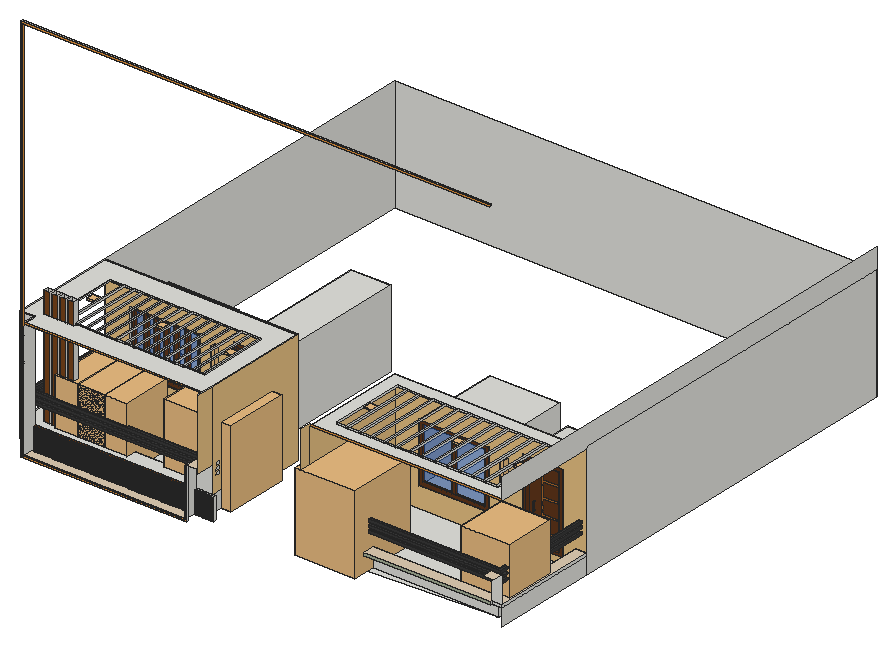
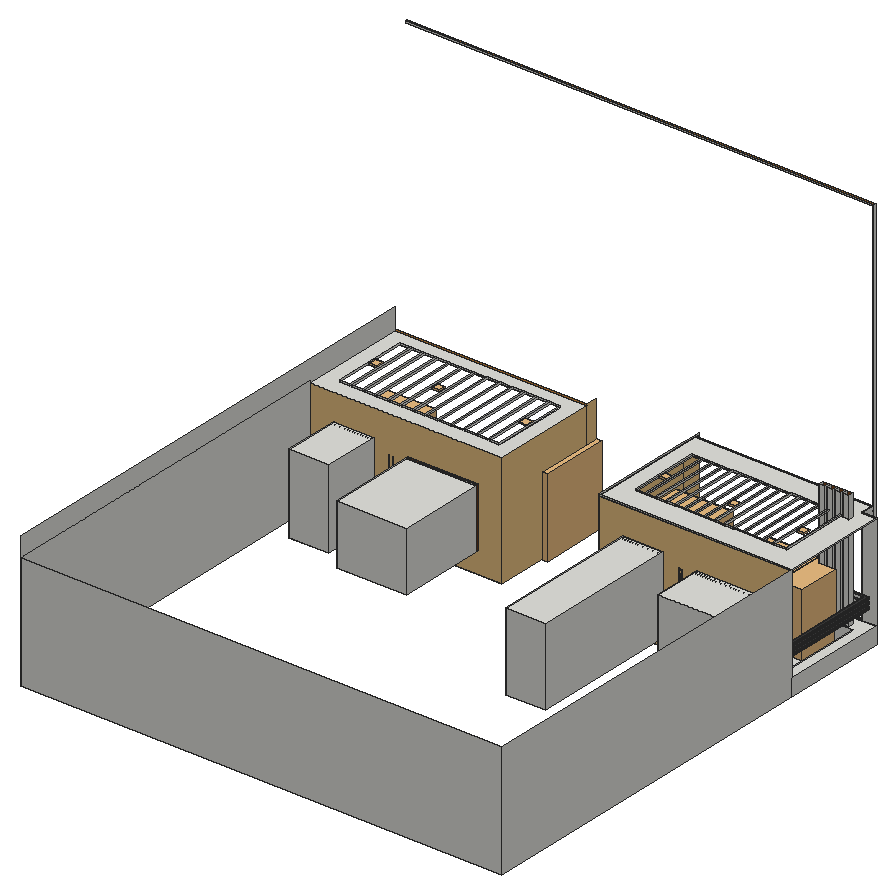
# SketchUp Ruby script. Lengths in inches.
U = 1.inch
M = Sketchup.active_model
def pt(a) = Geom::Point3d.new(a.map { |v| v * U })
def face(e, loops, mat)
  f = e.add_face(loops[0].map { |a| pt(a) })
  loops[1..].each { |l| e.add_face(l.map { |a| pt(a) }).erase! }
  f.material = f.back_material = mat if mat
  f
end
# faces: each face lists its corners as indices into pts; further lists are holes
def faces(e, pts, list, mat = nil) = list.each { |f| face(e, (f[0].is_a?(Array) ? f : [f]).map { |l| l.map { |i| pts[i] } }, mat) }
# xy, xz, yz: faces in a plane at the given z, y or x. An outline is a flat list of corners, or four numbers for a rectangle; further outlines are holes
def ring(l) = l.size == 4 ? [[l[0], l[1]], [l[2], l[1]], [l[2], l[3]], [l[0], l[3]]] : l.each_slice(2).to_a
def flat(e, list, mat, &to3) = list.each { |f| face(e, (f[0].is_a?(Array) ? f : [f]).map { |l| ring(l).map { |u, v| to3.(u, v) } }, mat) }
def xy(e, z, list, mat = nil) = flat(e, list, mat) { |x, y| [x, y, z] }
def xz(e, y, list, mat = nil) = flat(e, list, mat) { |x, z| [x, y, z] }
def yz(e, x, list, mat = nil) = flat(e, list, mat) { |y, z| [x, y, z] }
def lines(e, pts, list) = list.each { |a, b| e.add_line(pt(pts[a]), pt(pts[b])) }
# prism: a flat outline (further loops are holes) pulled along v
def prism(e, loops, v, mat = nil)
  f = face(e, loops, mat); d = Geom::Vector3d.new(v.map { |x| x * U })
  f.pushpull(f.normal.samedirection?(d) ? d.length : -d.length)
end
def box(e, o, s, mat = nil) = prism(e, [[o, [o[0] + s[0], o[1], o[2]], [o[0] + s[0], o[1] + s[1], o[2]], [o[0], o[1] + s[1], o[2]]]], [0, 0, s[2]], mat)
def at(x, y, z, deg = 0) = Geom::Transformation.translation(pt([x, y, z])) * Geom::Transformation.rotation(ORIGIN, Z_AXIS, deg.degrees)
def axes(o, x, y, z) = Geom::Transformation.new([*x, 0, *y, 0, *z, 0, *pt(o).to_a, 1])
def part(name) = M.definitions.add(name)
# library, detail: a bought-in or finely detailed component or shape, given as its bounding box
def library(name, o, s) = part(name).tap { |d| box(d.entities, o, s) }
def detail(e, o, s) = box(e.add_group.entities, o, s)
def put(e, d, t, mat = nil) = e.add_instance(d, t).tap { |i| i.material = mat if mat }
def group(e, t, mat = nil) = e.add_group.tap { |g| g.transformation = t; g.material = mat if mat }.entities
root = M.entities
M.materials.add("Generic\#1").color = [121, 68, 27]
M.materials.add("Generic\#4").color = [232, 149, 60]
M.materials.add("Generic\#5").color = [233, 194, 132]
M.materials.add("Generic\#6").color = [223, 205, 179]
M.materials.add("Generic\#8").color = [168, 180, 155]
M.materials.add("[Color M05]").color = [114, 114, 114]
M.materials.add("[Color M07]").color = [58, 58, 58]
M.materials.add("[Translucent Glass Blue]").color = [28, 83, 181]
M.materials["[Translucent Glass Blue]"].alpha = 0.5
M.materials.add("[Wood Bamboo]").color = [177, 105, 43]
M.materials.add("[Wood Cherry Original]").color = [96, 54, 26]
c1 = part("Group\#9")
xy(c1.entities,22.76,[[0,0,2,3]])
xz(c1.entities,0,[[0,0,2,22.76]])
yz(c1.entities,0,[[0,0,3,22.76]])
yz(c1.entities,2,[[0,0,3,22.76]])
c2 = library("Plant",[-27.84,-31.84,-1.26],[68.28,70.82,154.38])
c3 = library("Plant+2 (1)",[-9.13,-9.52,0],[51.76,51.77,66.88])
c4 = library("Flora+17",[-57.52,158.6,-38.64],[66.99,62.88,77.28])
c5 = part("Group\#5")
xy(c5.entities,0,[[0,0,41.8125,3.4375]],"[Wood Cherry Original]")
xy(c5.entities,3.53,[[3.53,0,38.28,3.4375]],"[Wood Cherry Original]")
xy(c5.entities,31.39,[[9.28,1.32,9.97,3.4375]])
xy(c5.entities,32.05,[[9.29,1.98,9.98,3.4375]],"[Color M05]")
xy(c5.entities,39.77,[[9.29,1.98,9.98,3.4375]])
xy(c5.entities,40.43,[[9.28,1.32,9.97,3.4375]],"[Color M05]")
xy(c5.entities,79.47,[[3.53,0,38.28,3.4375]],"[Wood Cherry Original]")
xy(c5.entities,83,[[0,0,41.8125,3.4375]],"[Wood Cherry Original]")
xz(c5.entities,0,[[[0,0,41.8125,83],[3.53,3.53,38.28,79.47]]],"[Wood Cherry Original]")
xz(c5.entities,1.32,[[9.28,31.39,9.97,40.43]],"[Color M05]")
xz(c5.entities,1.98,[[9.29,32.05,9.98,39.77]],"[Color M05]")
xz(c5.entities,3.4375,[[9.29,39.77,9.28,40.43,9.97,40.43,9.98,39.77]])
xz(c5.entities,3.4375,[[16.22,3.53,17.74,3.53,17.74,13.29,38.28,13.29,38.28,15.09,17.74,15.09,17.74,29.41,38.28,29.41,38.28,31.22,17.74,31.22,17.74,45.54,38.28,45.54,38.28,47.34,17.74,47.34,17.74,61.66,38.28,61.66,38.28,63.47,17.74,63.47,17.74,79.47,16.22,79.47]],"[Wood Bamboo]")
xz(c5.entities,3.4375,[[[0,0,41.8125,83],[3.53,3.53,38.28,79.47]],[[3.53,3.53,16.22,79.47],[9.29,39.77,9.28,40.43,9.97,40.43,9.98,39.77],[9.28,31.39,9.29,32.05,9.98,32.05,9.97,31.39]],[17.74,3.53,38.28,13.29],[17.74,15.09,38.28,29.41],[17.74,31.22,38.28,45.54],
  [17.74,47.34,38.28,61.66],[17.74,63.47,38.28,79.47]],"[Wood Cherry Original]")
yz(c5.entities,0,[[0,0,3.4375,83]],"[Wood Cherry Original]")
yz(c5.entities,3.53,[[0,3.53,3.4375,79.47]],"[Wood Cherry Original]")
yz(c5.entities,38.28,[[0,3.53,3.4375,79.47]],"[Wood Cherry Original]")
yz(c5.entities,41.8125,[[0,0,3.4375,83]],"[Wood Cherry Original]")
p = [[9.28,1.32,40.43],[9.29,1.98,39.77],[9.29,1.98,32.05],[9.28,1.32,31.39],[9.29,3.4375,32.05],[9.28,3.4375,31.39],
  [9.98,1.98,39.77],[9.97,1.32,40.43],[9.97,1.32,31.39],[9.98,1.98,32.05],[9.97,3.4375,31.39],[9.98,3.4375,32.05],
  [9.28,3.4375,40.43],[9.29,3.4375,39.77],[9.98,3.4375,39.77],[9.97,3.4375,40.43],[9.625,3.4375,40.13],[9.625,1.625,40.13],
  [9.625,1.625,31.69],[9.625,3.4375,31.69]]
faces(c5.entities,p,[[0,1,2,3],[3,2,4,5],[6,7,8,9],[9,8,10,11],[12,13,1,0],[14,15,7,6]],"[Color M05]")
lines(c5.entities,p,[[16,17],[18,19],[17,18]])
c6 = part("Group\#3")
xy(c6.entities,0,[[0,0,81.86,2.5]],"[Wood Cherry Original]")
xy(c6.entities,4.12,[[4.12,0,13.68,2.5],[13.68,0,18.93,2.5],[18.93,0,25.68,2.5],[25.68,0,30.93,2.5],[30.93,0,37.68,2.5],
  [37.68,0,42.93,2.5],[42.93,0,49.68,2.5],[49.68,0,54.93,2.5],[54.93,0,61.68,2.5],[61.68,0,66.93,2.5],
  [66.93,0,77.74,2.5]],"[Wood Cherry Original]")
xy(c6.entities,66.49,[[4.12,0,13.68,2.5],[13.68,0,18.93,2.5],[18.93,0,25.68,2.5],[25.68,0,30.93,2.5],[30.93,0,37.68,2.5],
  [37.68,0,42.93,2.5],[42.93,0,49.68,2.5],[49.68,0,54.93,2.5],[54.93,0,61.68,2.5],[61.68,0,66.93,2.5],
  [66.93,0,77.74,2.5]],"[Wood Cherry Original]")
xy(c6.entities,70.61,[[0,0,81.86,2.5]],"[Wood Cherry Original]")
xz(c6.entities,0,[[[0,0,81.86,70.61],[4.12,4.12,77.74,66.49]],[13.68,4.12,18.93,66.49],[25.68,4.12,30.93,66.49],[37.68,4.12,42.93,66.49],[49.68,4.12,54.93,66.49],
  [61.68,4.12,66.93,66.49]],"[Wood Cherry Original]")
xz(c6.entities,2.5,[[4.12,4.12,13.68,66.49],[18.93,4.12,25.68,66.49],[30.93,4.12,37.68,66.49],[42.93,4.12,49.68,66.49],[54.93,4.12,61.68,66.49],
  [66.93,4.12,77.74,66.49]],"[Translucent Glass Blue]")
xz(c6.entities,2.5,[[[0,0,81.86,70.61],[4.12,4.12,77.74,66.49]]],"[Wood Cherry Original]")
yz(c6.entities,0,[[0,0,2.5,70.61]],"[Wood Cherry Original]")
yz(c6.entities,4.12,[[0,4.12,2.5,66.49]],"[Wood Cherry Original]")
yz(c6.entities,13.68,[[0,4.12,2.5,66.49]],"[Wood Cherry Original]")
yz(c6.entities,18.93,[[0,4.12,2.5,66.49]],"[Wood Cherry Original]")
yz(c6.entities,25.68,[[0,4.12,2.5,66.49]],"[Wood Cherry Original]")
yz(c6.entities,30.93,[[0,4.12,2.5,66.49]],"[Wood Cherry Original]")
yz(c6.entities,37.68,[[0,4.12,2.5,66.49]],"[Wood Cherry Original]")
yz(c6.entities,42.93,[[0,4.12,2.5,66.49]],"[Wood Cherry Original]")
yz(c6.entities,49.68,[[0,4.12,2.5,66.49]],"[Wood Cherry Original]")
yz(c6.entities,54.93,[[0,4.12,2.5,66.49]],"[Wood Cherry Original]")
yz(c6.entities,61.68,[[0,4.12,2.5,66.49]],"[Wood Cherry Original]")
yz(c6.entities,66.93,[[0,4.12,2.5,66.49]],"[Wood Cherry Original]")
yz(c6.entities,77.74,[[0,4.12,2.5,66.49]],"[Wood Cherry Original]")
yz(c6.entities,81.86,[[0,0,2.5,70.61]],"[Wood Cherry Original]")
c7 = part("Group\#4")
xy(c7.entities,0,[[0,0,73.625,2.0625]],"[Wood Cherry Original]")
xy(c7.entities,3.98,[[35.0625,0,38.75,2.0625]])
xy(c7.entities,3.98,[[3.98,0,35.0625,2.0625],[38.75,0,69.64,2.0625]],"[Wood Cherry Original]")
xy(c7.entities,58.39,[[35.0625,0,38.75,2.0625]])
xy(c7.entities,58.39,[[3.98,0,35.0625,2.0625],[38.75,0,69.64,2.0625]],"[Wood Cherry Original]")
xy(c7.entities,62.375,[[0,0,73.625,2.0625]],"[Wood Cherry Original]")
xz(c7.entities,0,[[[0,0,73.625,62.375],[3.98,3.98,69.64,58.39]],[35.0625,3.98,38.75,58.39]],"[Wood Cherry Original]")
xz(c7.entities,2.0625,[[[0,0,73.625,62.375],[3.98,3.98,69.64,58.39]]])
xz(c7.entities,2.0625,[[3.98,3.98,35.0625,58.39],[38.75,3.98,69.64,58.39]],"[Translucent Glass Blue]")
yz(c7.entities,0,[[0,0,2.0625,62.375]],"[Wood Cherry Original]")
yz(c7.entities,3.98,[[0,3.98,2.0625,58.39]],"[Wood Cherry Original]")
yz(c7.entities,35.0625,[[0,3.98,2.0625,58.39]],"[Wood Cherry Original]")
yz(c7.entities,38.75,[[0,3.98,2.0625,58.39]],"[Wood Cherry Original]")
yz(c7.entities,69.64,[[0,3.98,2.0625,58.39]],"[Wood Cherry Original]")
yz(c7.entities,73.625,[[0,0,2.0625,62.375]],"[Wood Cherry Original]")
c8 = library("Lamp Wall Outdoor 94-02",[-1.89,-4.65,-3.17],[3.78,4.65,6.35])
c9 = library("Tlon Light 450 Ceiling 152 006",[-8.86,-8.86,-3.78],[17.72,17.72,3.56])
xy(root,133.9375,[[15.3125,39.5,189,41]])
xy(root,135.68,[[18.375,51.5625,20.375,54.5625]])
xy(root,135.68,[[17.125,39.5,187.19,41]],"Generic\#4")
xy(root,135.68,[[17.125,41,187.19,41,187.19,54.5625,20.375,54.5625,20.375,51.5625,18.375,51.5625,18.375,54.5625,17.125,54.5625]],"Generic\#6")
xy(root,140.875,[[306.09,54.5625,306.09,65.5625,496.1875,65.5625],[306.09,65.5625,496.1875,166.1875],[496.1875,65.5625,496.1875,166.1875,507.875,166.1875],[13.4375,71.3125,204.09,166.1875]])
xy(root,148.11,[[440.99,166.1875,482.8,225.0625]])
xy(root,148.65,[[137.36,166.1875,179.17,320.375]])
xy(root,158.4375,[[316.59,52.5625,318.59,54.5625],[318.59,52.5625,497.875,54.5625],[[2.3125,54.5625,204.09,54.5625,204.09,71.3125,13.4375,71.3125,13.4375,166.1875,2.3125,166.1875],[36.28,64.07,42.47,69.2],[27.85,64.07,34.03,69.2],[44.72,64.07,50.91,69.2],[19.41,64.07,25.6,69.2]],[306.09,54.5625,306.09,65.5625,496.1875,65.5625,496.1875,166.1875,507.875,166.1875,507.875,54.5625]])
xy(root,161.25,[[316.59,52.5625,497.875,52.5625,497.875,54.5625,507.875,54.5625,507.875,166.1875,496.1875,166.1875,496.1875,65.5625,306.09,65.5625,306.09,54.5625,316.59,54.5625]],"Generic\#6")
xy(root,162.59,[[27.78,166.1875,101.4,217.3125],[331.4,166.1875,405.03,260.1875]])
xy(root,174.54,[[6.99,59.18,6.99,166.1875,10.24,166.1875,10.24,62.43,204.09,62.43,204.09,59.18]],"[Color M07]")
xy(root,176.92,[[306.09,58.82,306.09,61.82,500.27,61.82,500.27,166.1875,503.27,166.1875,503.27,58.82]])
xy(root,177.29,[[6.99,59.18,204.09,59.18,204.09,62.43,10.24,62.43,10.24,166.1875,6.99,166.1875]],"[Color M07]")
xy(root,179.16,[[6.99,59.18,6.99,166.1875,10.24,166.1875,10.24,62.43,204.09,62.43,204.09,59.18]],"[Color M07]")
xy(root,179.49,[[306.09,58.82,503.27,58.82,503.27,166.1875,500.27,166.1875,500.27,61.82,306.09,61.82]],"[Color M07]")
xy(root,181.91,[[6.99,59.18,204.09,59.18,204.09,62.43,10.24,62.43,10.24,166.1875,6.99,166.1875]],"[Color M07]")
xy(root,182.11,[[306.09,58.82,306.09,61.82,500.27,61.82,500.27,166.1875,503.27,166.1875,503.27,58.82]])
xy(root,183.68,[[6.99,59.18,6.99,166.1875,10.24,166.1875,10.24,62.43,204.09,62.43,204.09,59.18]],"[Color M07]")
xy(root,184.67,[[306.09,58.82,503.27,58.82,503.27,166.1875,500.27,166.1875,500.27,61.82,306.09,61.82]],"[Color M07]")
xy(root,186.43,[[187.19,39.5,189,41]])
xy(root,186.43,[[187.19,41,204.09,54.5625]],"Generic\#6")
xy(root,186.43,[[6.99,59.18,204.09,59.18,204.09,62.43,10.24,62.43,10.24,166.1875,6.99,166.1875]],"[Color M07]")
xy(root,187.42,[[306.09,58.82,306.09,61.82,500.27,61.82,500.27,166.1875,503.27,166.1875,503.27,58.82]])
xy(root,189.99,[[497.875,43.625,507.875,54.5625]],"Generic\#6")
xy(root,189.99,[[306.09,58.82,503.27,58.82,503.27,166.1875,500.27,166.1875,500.27,61.82,306.09,61.82]],"[Color M07]")
xy(root,192.9375,[[306.09,43.625,316.59,54.5625]],"Generic\#6")
xy(root,224.97,[[27.78,166.1875,101.4,217.3125],[331.4,166.1875,405.03,260.1875]])
xy(root,229.99,[[137.36,166.1875,179.17,320.375]])
xy(root,231.11,[[440.99,166.1875,482.8,225.0625]])
xy(root,259.1875,[[[306.09,54.5625,507.875,166.1875],[320.02,70.49,491.95,150.26]],[320.02,70.49,322.02,150.26],[331.7,70.49,333.7,150.26],[344.89,70.49,346.89,150.26],[358.07,70.49,360.07,150.26],
  [371.26,70.49,373.26,150.26],[384.45,70.49,386.45,150.26],[397.64,70.49,399.64,150.26],[410.82,70.49,412.82,150.26],[424.01,70.49,426.01,150.26],
  [437.2,70.49,439.2,150.26],[450.39,70.49,452.39,150.26],[463.57,70.49,465.57,150.26],[476.76,70.49,478.76,150.26],[489.95,70.49,491.95,150.26]])
xy(root,259.6875,[[[17.125,41,17.125,54.5625,2.3125,54.5625,2.3125,166.1875,204.09,166.1875,204.09,41],[27.64,66.32,186.39,140.86]],[27.64,66.32,28.83,140.86],[40.89,66.32,42.89,140.86],[51.14,66.32,53.14,140.86],[61.39,66.32,63.39,140.86],
  [71.64,66.32,73.64,140.86],[81.89,66.32,83.89,140.86],[92.14,66.32,94.14,140.86],[102.39,66.32,104.39,140.86],[112.64,66.32,114.64,140.86],
  [122.89,66.32,124.89,140.86],[133.14,66.32,135.14,140.86],[143.39,66.32,145.39,140.86],[153.64,66.32,155.64,140.86],[163.89,66.32,165.89,140.86],
  [174.14,66.32,176.14,140.86],[184.39,66.32,186.39,140.86]])
xz(root,39.5,[[15.3125,133.9375,189,133.9375,189,186.43,187.19,186.43,187.19,135.68,17.125,135.68,17.125,542.625,507.875,542.625,507.875,544.65,15.3125,544.65]],"Generic\#4")
xz(root,41,[[15.3125,133.9375,15.3125,544.65,507.875,544.65,507.875,542.625,17.125,542.625,17.125,135.68,187.19,135.68,187.19,186.43,189,186.43,189,133.9375]])
xz(root,41,[[17.125,259.6875,204.09,260.875]],"Generic\#4")
xz(root,52.5625,[[316.59,158.4375,497.875,161.25]],"Generic\#8")
xz(root,54.5625,[[17.125,135.68,18.375,158.4375],[18.375,135.68,20.375,158.4375],[20.375,135.68,187.19,158.4375],[2.3125,140.875,17.125,158.4375],[2.3125,158.4375,17.125,259.6875],
  [187.19,158.4375,204.09,186.43],[306.09,158.4375,316.59,161.25],[497.875,158.4375,507.875,161.25],[306.09,161.25,316.59,192.9375],[497.875,161.25,507.875,189.99],
  [2.3125,259.6875,17.125,260.875]])
xz(root,54.5625,[[306.09,259.1875,507.875,260.875]],"Generic\#4")
xz(root,58.82,[[306.09,176.92,503.27,179.49],[306.09,182.11,503.27,184.67],[306.09,187.42,503.27,189.99]],"[Color M07]")
xz(root,59.18,[[6.99,174.54,204.09,177.29],[6.99,179.16,204.09,181.91],[6.99,183.68,204.09,186.43]],"[Color M07]")
xz(root,61.82,[[306.09,176.92,500.27,179.49],[306.09,182.11,500.27,184.67],[306.09,187.42,500.27,189.99]],"[Color M07]")
xz(root,62.43,[[10.24,174.54,204.09,177.29],[10.24,179.16,204.09,181.91],[10.24,183.68,204.09,186.43]])
xz(root,64.07,[[19.41,158.4375,25.6,281.75],[27.85,158.4375,34.03,281.75],[36.28,158.4375,42.47,281.75],[44.72,158.4375,50.91,281.75]],"Generic\#1")
xz(root,65.5625,[[306.09,140.875,496.1875,155.5],[306.09,155.5,496.1875,158.4375],[306.09,158.4375,496.1875,161.25]])
xz(root,66.32,[[27.64,259.6875,28.83,260.875],[28.83,259.6875,40.89,260.875],[40.89,259.6875,42.89,260.875],[42.89,259.6875,51.14,260.875],[51.14,259.6875,53.14,260.875],
  [53.14,259.6875,61.39,260.875],[61.39,259.6875,63.39,260.875],[63.39,259.6875,71.64,260.875],[71.64,259.6875,73.64,260.875],[73.64,259.6875,81.89,260.875],
  [81.89,259.6875,83.89,260.875],[83.89,259.6875,92.14,260.875],[92.14,259.6875,94.14,260.875],[94.14,259.6875,102.39,260.875],[102.39,259.6875,104.39,260.875],
  [104.39,259.6875,112.64,260.875],[112.64,259.6875,114.64,260.875],[114.64,259.6875,122.89,260.875],[122.89,259.6875,124.89,260.875],[124.89,259.6875,133.14,260.875],
  [133.14,259.6875,135.14,260.875],[135.14,259.6875,143.39,260.875],[143.39,259.6875,145.39,260.875],[145.39,259.6875,153.64,260.875],[153.64,259.6875,155.64,260.875],
  [155.64,259.6875,163.89,260.875],[163.89,259.6875,165.89,260.875],[165.89,259.6875,174.14,260.875],[174.14,259.6875,176.14,260.875],[176.14,259.6875,184.39,260.875],
  [184.39,259.6875,186.39,260.875]])
xz(root,69.2,[[19.41,158.4375,25.6,281.75],[27.85,158.4375,34.03,281.75],[36.28,158.4375,42.47,281.75],[44.72,158.4375,50.91,281.75]])
xz(root,70.49,[[322.02,259.1875,331.7,260.875],[333.7,259.1875,344.89,260.875],[346.89,259.1875,358.07,260.875],[360.07,259.1875,371.26,260.875],[373.26,259.1875,384.45,260.875],
  [386.45,259.1875,397.64,260.875],[399.64,259.1875,410.82,260.875],[412.82,259.1875,424.01,260.875],[426.01,259.1875,437.2,260.875],[439.2,259.1875,450.39,260.875],
  [452.39,259.1875,463.57,260.875],[465.57,259.1875,476.76,260.875],[478.76,259.1875,489.95,260.875]])
xz(root,71.3125,[[13.4375,140.875,204.09,158.4375]])
xz(root,140.86,[[27.64,259.6875,28.83,260.875],[28.83,259.6875,40.89,260.875],[40.89,259.6875,42.89,260.875],[42.89,259.6875,51.14,260.875],[51.14,259.6875,53.14,260.875],
  [53.14,259.6875,61.39,260.875],[61.39,259.6875,63.39,260.875],[63.39,259.6875,71.64,260.875],[71.64,259.6875,73.64,260.875],[73.64,259.6875,81.89,260.875],
  [81.89,259.6875,83.89,260.875],[83.89,259.6875,92.14,260.875],[92.14,259.6875,94.14,260.875],[94.14,259.6875,102.39,260.875],[102.39,259.6875,104.39,260.875],
  [104.39,259.6875,112.64,260.875],[112.64,259.6875,114.64,260.875],[114.64,259.6875,122.89,260.875],[122.89,259.6875,124.89,260.875],[124.89,259.6875,133.14,260.875],
  [133.14,259.6875,135.14,260.875],[135.14,259.6875,143.39,260.875],[143.39,259.6875,145.39,260.875],[145.39,259.6875,153.64,260.875],[153.64,259.6875,155.64,260.875],
  [155.64,259.6875,163.89,260.875],[163.89,259.6875,165.89,260.875],[165.89,259.6875,174.14,260.875],[174.14,259.6875,176.14,260.875],[176.14,259.6875,184.39,260.875],
  [184.39,259.6875,186.39,260.875]])
xz(root,150.26,[[322.02,259.1875,331.7,260.875],[333.7,259.1875,344.89,260.875],[346.89,259.1875,358.07,260.875],[360.07,259.1875,371.26,260.875],[373.26,259.1875,384.45,260.875],
  [386.45,259.1875,397.64,260.875],[399.64,259.1875,410.82,260.875],[412.82,259.1875,424.01,260.875],[426.01,259.1875,437.2,260.875],[439.2,259.1875,450.39,260.875],
  [452.39,259.1875,463.57,260.875],[465.57,259.1875,476.76,260.875],[478.76,259.1875,489.95,260.875]])
xz(root,166.1875,[[496.1875,158.4375,507.875,161.25],[2.3125,259.6875,204.09,260.875]])
xz(root,166.1875,[[[13.4375,140.875,204.09,140.875,204.09,259.6875,2.3125,259.6875,2.3125,158.4375,13.4375,158.4375],[27.78,162.59,101.4,224.97],[137.36,148.65,179.17,229.99],[6.99,183.68,10.24,186.43],[6.99,179.16,10.24,181.91],[6.99,174.54,10.24,177.29]],[[306.09,140.875,496.1875,140.875,496.1875,161.25,507.875,161.25,507.875,259.1875,306.09,259.1875],[331.4,162.59,405.03,224.97],[440.99,148.11,482.8,231.11],[500.27,176.92,503.27,179.49],[500.27,182.11,503.27,184.67],[500.27,187.42,503.27,189.99]]],"Generic\#5")
xz(root,217.3125,[[27.78,162.59,101.4,224.97]])
xz(root,225.0625,[[440.99,148.11,482.8,231.11]])
xz(root,260.1875,[[331.4,162.59,405.03,224.97]])
xz(root,320.375,[[137.36,148.65,179.17,229.99]])
xz(root,546.8125,[[2.3125,140.875,507.875,260.875]])
yz(root,2.3125,[[54.5625,140.875,166.1875,158.4375],[166.1875,140.875,546.8125,260.875],[54.5625,259.6875,166.1875,260.875]])
yz(root,6.99,[[59.18,174.54,166.1875,177.29],[59.18,179.16,166.1875,181.91],[59.18,183.68,166.1875,186.43]],"[Color M07]")
yz(root,10.24,[[62.43,174.54,166.1875,177.29],[62.43,179.16,166.1875,181.91],[62.43,183.68,166.1875,186.43]],"[Color M07]")
yz(root,13.4375,[[71.3125,140.875,166.1875,158.4375]])
yz(root,15.3125,[[39.5,133.9375,41,544.65]])
yz(root,17.125,[[41,135.68,54.5625,259.6875],[41,259.6875,54.5625,260.875]])
yz(root,17.125,[[39.5,135.68,41,542.625]],"Generic\#4")
yz(root,19.41,[[64.07,158.4375,69.2,281.75]])
yz(root,25.6,[[64.07,158.4375,69.2,281.75]])
yz(root,27.64,[[66.32,259.6875,79.89,260.875],[79.89,259.6875,140.86,260.875]])
yz(root,27.78,[[166.1875,162.59,217.3125,224.97]])
yz(root,27.85,[[64.07,158.4375,69.2,281.75]])
yz(root,28.83,[[66.32,259.6875,140.86,260.875]])
yz(root,34.03,[[64.07,158.4375,69.2,281.75]])
yz(root,36.28,[[64.07,158.4375,69.2,281.75]])
yz(root,40.89,[[66.32,259.6875,140.86,260.875]])
yz(root,42.47,[[64.07,158.4375,69.2,281.75]])
yz(root,42.89,[[66.32,259.6875,140.86,260.875]])
yz(root,44.72,[[64.07,158.4375,69.2,281.75]])
yz(root,50.91,[[64.07,158.4375,69.2,281.75]])
yz(root,51.14,[[66.32,259.6875,140.86,260.875]])
yz(root,53.14,[[66.32,259.6875,140.86,260.875]])
yz(root,61.39,[[66.32,259.6875,140.86,260.875]])
yz(root,63.39,[[66.32,259.6875,140.86,260.875]])
yz(root,71.64,[[66.32,259.6875,140.86,260.875]])
yz(root,73.64,[[66.32,259.6875,140.86,260.875]])
yz(root,81.89,[[66.32,259.6875,140.86,260.875]])
yz(root,83.89,[[66.32,259.6875,140.86,260.875]])
yz(root,92.14,[[66.32,259.6875,140.86,260.875]])
yz(root,94.14,[[66.32,259.6875,140.86,260.875]])
yz(root,101.4,[[166.1875,162.59,217.3125,224.97]])
yz(root,102.39,[[66.32,259.6875,140.86,260.875]])
yz(root,104.39,[[66.32,259.6875,140.86,260.875]])
yz(root,112.64,[[66.32,259.6875,140.86,260.875]])
yz(root,114.64,[[66.32,259.6875,140.86,260.875]])
yz(root,122.89,[[66.32,259.6875,140.86,260.875]])
yz(root,124.89,[[66.32,259.6875,140.86,260.875]])
yz(root,133.14,[[66.32,259.6875,140.86,260.875]])
yz(root,135.14,[[66.32,259.6875,140.86,260.875]])
yz(root,137.36,[[166.1875,148.65,320.375,229.99]])
yz(root,143.39,[[66.32,259.6875,140.86,260.875]])
yz(root,145.39,[[66.32,259.6875,140.86,260.875]])
yz(root,153.64,[[66.32,259.6875,140.86,260.875]])
yz(root,155.64,[[66.32,259.6875,140.86,260.875]])
yz(root,163.89,[[66.32,259.6875,140.86,260.875]])
yz(root,165.89,[[66.32,259.6875,140.86,260.875]])
yz(root,174.14,[[66.32,259.6875,140.86,260.875]])
yz(root,176.14,[[66.32,259.6875,140.86,260.875]])
yz(root,179.17,[[166.1875,148.65,320.375,229.99]])
yz(root,184.39,[[66.32,259.6875,140.86,260.875]])
yz(root,186.39,[[66.32,259.6875,140.86,260.875]])
yz(root,187.19,[[41,135.68,54.5625,186.43]])
yz(root,187.19,[[39.5,135.68,41,186.43]],"Generic\#4")
yz(root,189,[[39.5,133.9375,41,186.43]])
yz(root,204.09,[[54.5625,140.875,71.3125,158.4375],[59.18,174.54,62.43,177.29],[59.18,179.16,62.43,181.91],[59.18,183.68,62.43,186.43],[35.5625,259.6875,41,260.875],
  [41,259.6875,54.5625,260.875],[54.5625,259.6875,166.1875,260.875]])
yz(root,204.09,[[[71.3125,140.875,71.3125,158.4375,54.5625,158.4375,54.5625,259.6875,166.1875,259.6875,166.1875,140.875],[59.18,183.68,62.43,186.43],[59.18,179.16,62.43,181.91],[59.18,174.54,62.43,177.29]],[35.5625,186.43,54.5625,259.6875]],"Generic\#5")
yz(root,306.09,[[54.5625,140.875,65.5625,158.4375],[54.5625,158.4375,65.5625,161.25],[58.82,176.92,61.82,179.49],[58.82,182.11,61.82,184.67],[58.82,187.42,61.82,189.99]])
yz(root,306.09,[[[65.5625,140.875,166.1875,140.875,166.1875,259.1875,54.5625,259.1875,54.5625,161.25,65.5625,161.25],[58.82,187.42,61.82,189.99],[58.82,182.11,61.82,184.67],[58.82,176.92,61.82,179.49]],[43.625,192.9375,54.5625,260.875]],"Generic\#5")
yz(root,316.59,[[52.5625,158.4375,54.5625,161.25]])
yz(root,322.02,[[70.49,259.1875,150.26,260.875]])
yz(root,331.4,[[166.1875,162.59,260.1875,224.97]])
yz(root,331.7,[[70.49,259.1875,150.26,260.875]])
yz(root,333.7,[[70.49,259.1875,150.26,260.875]])
yz(root,344.89,[[70.49,259.1875,150.26,260.875]])
yz(root,346.89,[[70.49,259.1875,150.26,260.875]])
yz(root,358.07,[[70.49,259.1875,150.26,260.875]])
yz(root,360.07,[[70.49,259.1875,150.26,260.875]])
yz(root,371.26,[[70.49,259.1875,150.26,260.875]])
yz(root,373.26,[[70.49,259.1875,150.26,260.875]])
yz(root,384.45,[[70.49,259.1875,150.26,260.875]])
yz(root,386.45,[[70.49,259.1875,150.26,260.875]])
yz(root,397.64,[[70.49,259.1875,150.26,260.875]])
yz(root,399.64,[[70.49,259.1875,150.26,260.875]])
yz(root,405.03,[[166.1875,162.59,260.1875,224.97]])
yz(root,410.82,[[70.49,259.1875,150.26,260.875]])
yz(root,412.82,[[70.49,259.1875,150.26,260.875]])
yz(root,424.01,[[70.49,259.1875,150.26,260.875]])
yz(root,426.01,[[70.49,259.1875,150.26,260.875]])
yz(root,437.2,[[70.49,259.1875,150.26,260.875]])
yz(root,439.2,[[70.49,259.1875,150.26,260.875]])
yz(root,440.99,[[166.1875,148.11,225.0625,231.11]])
yz(root,450.39,[[70.49,259.1875,150.26,260.875]])
yz(root,452.39,[[70.49,259.1875,150.26,260.875]])
yz(root,463.57,[[70.49,259.1875,150.26,260.875]])
yz(root,465.57,[[70.49,259.1875,150.26,260.875]])
yz(root,476.76,[[70.49,259.1875,150.26,260.875]])
yz(root,478.76,[[70.49,259.1875,150.26,260.875]])
yz(root,482.8,[[166.1875,148.11,225.0625,231.11]])
yz(root,489.95,[[70.49,259.1875,150.26,260.875]])
yz(root,496.1875,[[65.5625,140.875,166.1875,158.4375],[65.5625,158.4375,166.1875,161.25]])
yz(root,497.875,[[52.5625,158.4375,54.5625,161.25]])
yz(root,500.27,[[61.82,176.92,166.1875,179.49],[61.82,182.11,166.1875,184.67],[61.82,187.42,166.1875,189.99]],"[Color M07]")
yz(root,503.27,[[58.82,176.92,166.1875,179.49],[58.82,182.11,166.1875,184.67],[58.82,187.42,166.1875,189.99]],"[Color M07]")
yz(root,507.875,[[54.5625,140.875,166.1875,158.4375],[166.1875,140.875,546.8125,260.875],[54.5625,158.4375,166.1875,161.25],[54.5625,259.1875,166.1875,259.1875,166.1875,260.875,546.8125,260.875,546.8125,281.75,54.5625,281.75]])
p = [[2.3125,166.1875,140.875],[13.4375,166.1875,140.875],[306.09,60.0625,178.1875],[502.03,60.0625,178.1875],[306.09,60.0625,183.5],[502.03,60.0625,183.5],
  [502.03,166.1875,183.5],[306.09,60.0625,188.8125],[502.03,60.0625,188.8125],[502.03,166.1875,188.8125],[502.03,166.1875,178.1875],[204.09,60.0625,175.75],
  [7.875,60.0625,175.75],[7.875,166.1875,175.75],[7.875,166.1875,180.5],[7.875,60.0625,180.5],[204.09,60.0625,180.5],[7.875,166.1875,185],
  [7.875,60.0625,185],[204.09,60.0625,185]]
lines(root,p,[[0,1],[2,3],[4,5],[6,5],[7,8],[9,8],[10,3],[11,12],[13,12],[14,15],[16,15],[17,18],
  [19,18]])
put(root,c1,at(18.375,51.5625,135.68),"Generic\#1")
put(root,c1,at(21.25,51.5625,135.68),"Generic\#1")
put(root,c1,at(24.125,51.5625,135.68),"Generic\#1")
put(root,c1,at(27,51.5625,135.68),"Generic\#1")
put(root,c1,at(29.875,51.5625,135.68),"Generic\#1")
put(root,c1,at(32.75,51.5625,135.68),"Generic\#1")
put(root,c1,at(35.625,51.5625,135.68),"Generic\#1")
put(root,c1,at(38.5,51.5625,135.68),"Generic\#1")
put(root,c1,at(41.375,51.5625,135.68),"Generic\#1")
put(root,c1,at(44.25,51.5625,135.68),"Generic\#1")
put(root,c1,at(47.125,51.5625,135.68),"Generic\#1")
put(root,c1,at(50,51.5625,135.68),"Generic\#1")
put(root,c1,at(52.875,51.5625,135.68),"Generic\#1")
put(root,c1,at(55.75,51.5625,135.68),"Generic\#1")
put(root,c1,at(58.625,51.5625,135.68),"Generic\#1")
put(root,c1,at(61.5,51.5625,135.68),"Generic\#1")
put(root,c1,at(64.375,51.5625,135.68),"Generic\#1")
put(root,c1,at(67.25,51.5625,135.68),"Generic\#1")
put(root,c1,at(70.125,51.5625,135.68),"Generic\#1")
put(root,c1,at(73,51.5625,135.68),"Generic\#1")
put(root,c1,at(75.875,51.5625,135.68),"Generic\#1")
put(root,c1,at(78.75,51.5625,135.68),"Generic\#1")
put(root,c1,at(81.625,51.5625,135.68),"Generic\#1")
put(root,c1,at(84.5,51.5625,135.68),"Generic\#1")
put(root,c1,at(87.375,51.5625,135.68),"Generic\#1")
put(root,c1,at(90.25,51.5625,135.68),"Generic\#1")
put(root,c1,at(93.125,51.5625,135.68),"Generic\#1")
put(root,c1,at(96,51.5625,135.68),"Generic\#1")
put(root,c1,at(98.875,51.5625,135.68),"Generic\#1")
put(root,c1,at(101.75,51.5625,135.68),"Generic\#1")
put(root,c1,at(104.625,51.5625,135.68),"Generic\#1")
put(root,c1,at(107.5,51.5625,135.68),"Generic\#1")
put(root,c1,at(110.375,51.5625,135.68),"Generic\#1")
put(root,c1,at(113.25,51.5625,135.68),"Generic\#1")
put(root,c1,at(116.125,51.5625,135.68),"Generic\#1")
put(root,c1,at(119,51.5625,135.68),"Generic\#1")
put(root,c1,at(121.875,51.5625,135.68),"Generic\#1")
put(root,c1,at(124.75,51.5625,135.68),"Generic\#1")
put(root,c1,at(127.625,51.5625,135.68),"Generic\#1")
put(root,c1,at(130.5,51.5625,135.68),"Generic\#1")
put(root,c1,at(133.375,51.5625,135.68),"Generic\#1")
put(root,c1,at(136.25,51.5625,135.68),"Generic\#1")
put(root,c1,at(139.125,51.5625,135.68),"Generic\#1")
put(root,c1,at(142,51.5625,135.68),"Generic\#1")
put(root,c1,at(144.875,51.5625,135.68),"Generic\#1")
put(root,c1,at(147.75,51.5625,135.68),"Generic\#1")
put(root,c1,at(150.8125,51.5625,135.68),"Generic\#1")
put(root,c1,at(153.875,51.5625,135.68),"Generic\#1")
put(root,c1,at(156.9375,51.5625,135.68),"Generic\#1")
put(root,c1,at(160,51.5625,135.68),"Generic\#1")
put(root,c1,at(163.0625,51.5625,135.68),"Generic\#1")
put(root,c1,at(166.125,51.5625,135.68),"Generic\#1")
put(root,c1,at(169.1875,51.5625,135.68),"Generic\#1")
put(root,c1,at(172.25,51.5625,135.68),"Generic\#1")
put(root,c1,at(175.3125,51.5625,135.68),"Generic\#1")
put(root,c1,at(178.375,51.5625,135.68),"Generic\#1")
put(root,c1,at(181.4375,51.5625,135.68),"Generic\#1")
put(root,c1,at(184.5,51.5625,135.68),"Generic\#1")
put(root,c1,at(187.5625,51.5625,135.68))
put(root,c1,at(190.625,51.5625,135.68))
put(root,c1,at(193.6875,51.5625,135.68))
put(root,c1,at(196.75,51.5625,135.68))
put(root,c1,at(199.8125,51.5625,135.68))
put(root,c1,at(202.875,51.5625,135.68))
put(root,c1,at(205.9375,51.5625,135.68))
put(root,c2,axes([474.87,92.49,140.19],[0.7475,0,0],[0,0.7475,0],[0,0,0.46087]))
put(root,c3,at(66.45,71.11,140.875))
put(root,c3,at(42.57,71.11,140.875))
put(root,c3,axes([311.4,55.49,140.875],[1.23,0,0],[0,1.3899,0],[0,0,1.23]))
put(root,c4,axes([204.51,-100.25,181.45],[1.05,0,0],[0,1.05,0],[0,0,1.05]))
put(root,c5,at(440.99,166.1875,148.11))
put(root,c5,axes([137.36,166.1875,148.65],[1,0,0],[0,1,0],[0,0,0.98]))
put(root,c6,axes([27.78,168.92,162.72],[0.89936,0,0],[0,0.8633,0],[0,0,0.88057]))
put(root,c7,at(331.38,166.23,163.5))
put(root,c8,axes([118.9,166.1875,210.3],[1,0,0],[0,1,0],[0,0,3.19]))
put(root,c8,axes([422.9,166.1875,210.3],[1,0,0],[0,1,0],[0,0,3.19]))
put(root,c9,axes([484.55,108.73,261.2],[0.44852,0,0],[0,0.44852,0],[0,0,0.44852]))
put(root,c9,axes([418.98,108.73,261.2],[0.44852,0,0],[0,0.44852,0],[0,0,0.44852]))
put(root,c9,axes([327.17,108.73,261.2],[0.44852,0,0],[0,0.44852,0],[0,0,0.44852]))
put(root,c9,axes([180.36,108.73,261.2],[0.44852,0,0],[0,0.44852,0],[0,0,0.44852]))
put(root,c9,axes([108.37,108.73,261.2],[0.44852,0,0],[0,0.44852,0],[0,0,0.44852]))
put(root,c9,axes([35.8,108.73,261.2],[0.44852,0,0],[0,0.44852,0],[0,0,0.44852]))
